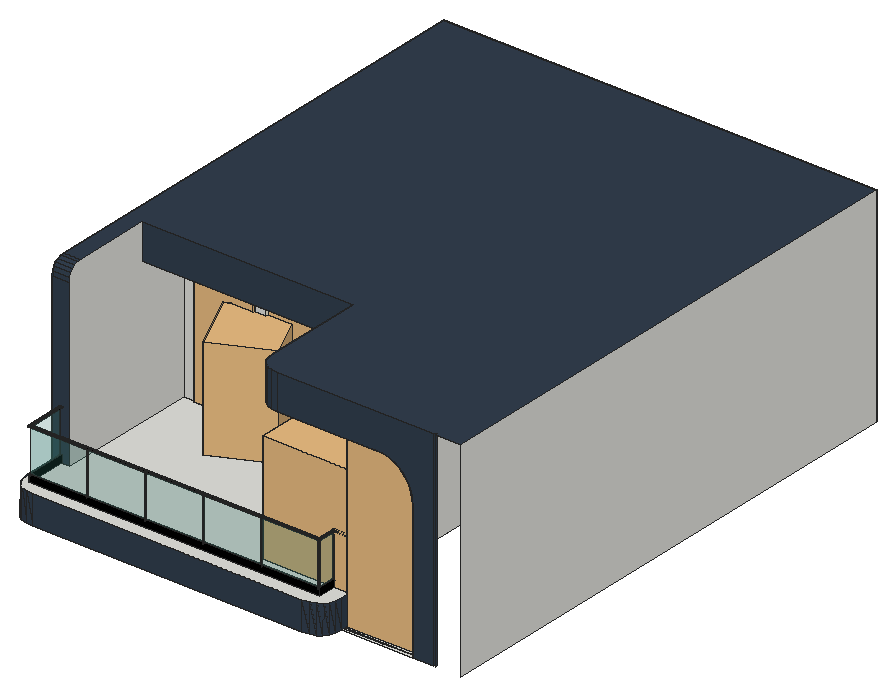
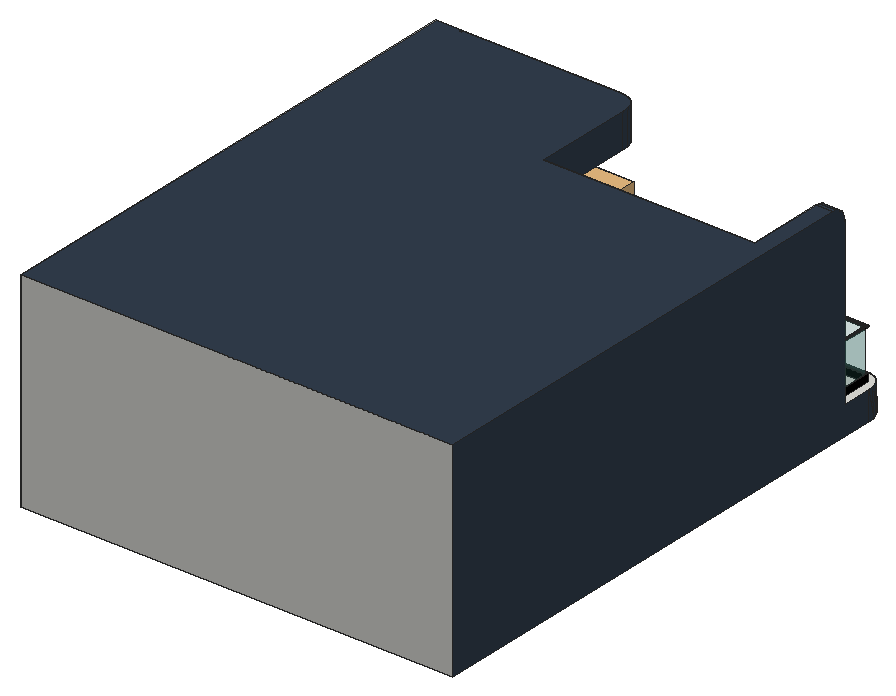
# SketchUp Ruby script. Lengths in inches.
U = 1.inch
M = Sketchup.active_model
def pt(a) = Geom::Point3d.new(a.map { |v| v * U })
def face(e, loops, mat)
  f = e.add_face(loops[0].map { |a| pt(a) })
  loops[1..].each { |l| e.add_face(l.map { |a| pt(a) }).erase! }
  f.material = f.back_material = mat if mat
  f
end
# faces: each face lists its corners as indices into pts; further lists are holes
def faces(e, pts, list, mat = nil) = list.each { |f| face(e, (f[0].is_a?(Array) ? f : [f]).map { |l| l.map { |i| pts[i] } }, mat) }
# xy, xz, yz: faces in a plane at the given z, y or x. An outline is a flat list of corners, or four numbers for a rectangle; further outlines are holes
def ring(l) = l.size == 4 ? [[l[0], l[1]], [l[2], l[1]], [l[2], l[3]], [l[0], l[3]]] : l.each_slice(2).to_a
def flat(e, list, mat, &to3) = list.each { |f| face(e, (f[0].is_a?(Array) ? f : [f]).map { |l| ring(l).map { |u, v| to3.(u, v) } }, mat) }
def xy(e, z, list, mat = nil) = flat(e, list, mat) { |x, y| [x, y, z] }
def xz(e, y, list, mat = nil) = flat(e, list, mat) { |x, z| [x, y, z] }
def yz(e, x, list, mat = nil) = flat(e, list, mat) { |y, z| [x, y, z] }
def lines(e, pts, list) = list.each { |a, b| e.add_line(pt(pts[a]), pt(pts[b])) }
# prism: a flat outline (further loops are holes) pulled along v
def prism(e, loops, v, mat = nil)
  f = face(e, loops, mat); d = Geom::Vector3d.new(v.map { |x| x * U })
  f.pushpull(f.normal.samedirection?(d) ? d.length : -d.length)
end
def box(e, o, s, mat = nil) = prism(e, [[o, [o[0] + s[0], o[1], o[2]], [o[0] + s[0], o[1] + s[1], o[2]], [o[0], o[1] + s[1], o[2]]]], [0, 0, s[2]], mat)
def at(x, y, z, deg = 0) = Geom::Transformation.translation(pt([x, y, z])) * Geom::Transformation.rotation(ORIGIN, Z_AXIS, deg.degrees)
def axes(o, x, y, z) = Geom::Transformation.new([*x, 0, *y, 0, *z, 0, *pt(o).to_a, 1])
def part(name) = M.definitions.add(name)
# library, detail: a bought-in or finely detailed component or shape, given as its bounding box
def library(name, o, s) = part(name).tap { |d| box(d.entities, o, s) }
def detail(e, o, s) = box(e.add_group.entities, o, s)
def put(e, d, t, mat = nil) = e.add_instance(d, t).tap { |i| i.material = mat if mat }
def group(e, t, mat = nil) = e.add_group.tap { |g| g.transformation = t; g.material = mat if mat }.entities
root = M.entities
M.materials.add("0399 AP 9182 LOST BLUE").color = [86, 115, 133]
M.materials.add("0400 AP 7301 PLUTO").color = [50, 63, 78]
M.materials.add("0897 AP 7835 CREAM CARESS").color = [247, 240, 216]
M.materials.add("Glass Railing Color").color = [198, 198, 198]
M.materials.add("Railing Glass").color = [63, 150, 137]
M.materials["Railing Glass"].alpha = 0.13
M.materials.add("[Color M09]").color = [0, 0, 0]
M.materials.add("[Wood Cherry Original]").color = [152, 86, 42]
M.materials.add("ground1").color = [30, 21, 16]
c1 = library("Group45\#2",[-24.46,-60,0],[48.92,120,0.375])
c2 = library("Cay chuoi",[-26.05,-21.66,0],[63.57,52.43,69.02])
c3 = library("door by lz",[5.91,-4.92,0],[35.43,6.61,78.74])
c4 = library("Спалня Венид",[0.07,-0.07,0],[84.71,86.8,39])
c5 = part("Glass Rail Spacer")
box(c5.entities,[-0.5,-0.25,0],[1,0.5,1],"Glass Railing Color")
c6 = part("Group97\#1")
xz(c6.entities,0,[[0.01,0,-0.18,0.02,-0.37,0.09,-0.52,0.21,-0.64,0.37,-0.72,0.54,-0.75,0.74,-0.73,0.93,-0.66,1.12,-0.54,1.27,-0.38,1.39,-0.21,1.47,-0.01,1.5,0.18,1.48,0.37,1.41,0.52,1.29,0.64,1.13,0.72,0.96,0.75,0.76,0.73,0.57,0.66,0.38,0.54,0.23,0.38,0.11,0.21,0.03]],"[Color M09]")
yz(c6.entities,212.09,[[-14.55,0,-14.36,0.03,-14.18,0.11,-14.02,0.23,-13.91,0.38,-13.84,0.57,-13.8125,0.76,-13.84,0.96,-13.92,1.13,-14.04,1.29,-14.2,1.41,-14.38,1.48,-14.57,1.5,-14.77,1.47,-14.95,1.39,-15.1,1.27,-15.22,1.12,-15.29,0.93,-15.3125,0.74,-15.28,0.54,-15.21,0.37,-15.08,0.21,-14.93,0.09,-14.75,0.02]],"[Color M09]")
p = [[-0.18,0,0.02],[-0.18,-27.5,0.02],[-0.37,-27.68,0.09],[-0.37,0,0.09],[200.81,-27.5,0.02],[200.99,-27.68,0.09],
  [200.81,-14.75,0.02],[200.99,-14.93,0.09],[0.01,0,0],[0.01,-27.3,0],[200.61,-27.3,0],[200.61,-14.55,0],
  [0.21,0,0.03],[0.21,-27.11,0.03],[200.42,-27.11,0.03],[200.42,-14.36,0.03],[0.38,0,0.11],[0.38,-26.93,0.11],
  [200.24,-26.93,0.11],[200.24,-14.18,0.11],[212.09,-14.75,0.02],[212.09,-14.93,0.09],[212.09,-14.55,0],[212.09,-14.36,0.03],
  [212.09,-14.18,0.11],[-0.52,-27.83,0.21],[-0.52,0,0.21],[201.15,-27.83,0.21],[201.15,-15.08,0.21],[0.54,0,0.23],
  [0.54,-26.77,0.23],[200.09,-26.77,0.23],[200.09,-14.02,0.23],[212.09,-15.08,0.21],[212.09,-14.02,0.23],[-0.64,-27.96,0.37],
  [-0.64,0,0.37],[201.27,-27.96,0.37],[201.27,-15.21,0.37],[0.66,0,0.38],[0.66,-26.66,0.38],[199.97,-26.66,0.38],
  [199.97,-13.91,0.38],[212.09,-15.21,0.37],[212.09,-13.91,0.38],[-0.72,-28.03,0.54],[-0.72,0,0.54],[201.35,-28.03,0.54],
  [201.35,-15.28,0.54],[0.73,0,0.57],[0.73,-26.59,0.57],[199.9,-26.59,0.57],[199.9,-13.84,0.57],[212.09,-15.28,0.54],
  [212.09,-13.84,0.57],[-0.75,-28.0625,0.74],[-0.75,0,0.74],[201.375,-28.0625,0.74],[201.375,-15.3125,0.74],[212.09,-15.3125,0.74],
  [0.75,0,0.76],[0.75,-26.5625,0.76],[199.875,-26.5625,0.76],[199.875,-13.8125,0.76],[212.09,-13.8125,0.76],[-0.73,-28.04,0.93],
  [-0.73,0,0.93],[201.35,-28.04,0.93],[201.35,-15.29,0.93],[212.09,-15.29,0.93],[0.72,0,0.96],[0.72,-26.59,0.96],
  [199.9,-26.59,0.96],[199.9,-13.84,0.96],[212.09,-13.84,0.96],[-0.66,-27.97,1.12],[-0.66,0,1.12],[201.28,-27.97,1.12],
  [201.28,-15.22,1.12],[212.09,-15.22,1.12],[0.64,0,1.13],[0.64,-26.67,1.13],[199.98,-26.67,1.13],[199.98,-13.92,1.13],
  [212.09,-13.92,1.13],[-0.54,-27.85,1.27],[-0.54,0,1.27],[201.16,-27.85,1.27],[201.16,-15.1,1.27],[0.52,0,1.29],
  [0.52,-26.79,1.29],[200.1,-26.79,1.29],[200.1,-14.04,1.29],[212.09,-15.1,1.27],[212.09,-14.04,1.29],[-0.38,-27.7,1.39],
  [-0.38,0,1.39],[201.01,-27.7,1.39],[201.01,-14.95,1.39],[0.37,0,1.41],[0.37,-26.95,1.41],[200.26,-26.95,1.41],
  [200.26,-14.2,1.41],[212.09,-14.95,1.39],[212.09,-14.2,1.41],[-0.21,-27.52,1.47],[-0.21,0,1.47],[200.83,-27.52,1.47],
  [200.83,-14.77,1.47],[0.18,0,1.48],[0.18,-27.13,1.48],[200.44,-27.13,1.48],[200.44,-14.38,1.48],[212.09,-14.77,1.47],
  [212.09,-14.38,1.48],[-0.01,-27.32,1.5],[-0.01,0,1.5],[200.64,-27.32,1.5],[200.64,-14.57,1.5],[212.09,-14.57,1.5]]
faces(c6.entities,p,[[0,1,2,3],[1,4,5,2],[4,6,7,5],[8,9,1,0],[9,10,4,1],[10,11,6,4],[12,13,9,8],[13,14,10,9],
  [14,15,11,10],[16,17,13,12],[17,18,14,13],[18,19,15,14],[6,20,21,7],[11,22,20,6],[15,23,22,11],[19,24,23,15],
  [3,2,25,26],[2,5,27,25],[5,7,28,27],[29,30,17,16],[30,31,18,17],[31,32,19,18],[7,21,33,28],[32,34,24,19],
  [26,25,35,36],[25,27,37,35],[27,28,38,37],[39,40,30,29],[40,41,31,30],[41,42,32,31],[28,33,43,38],[42,44,34,32],
  [36,35,45,46],[35,37,47,45],[37,38,48,47],[49,50,40,39],[50,51,41,40],[51,52,42,41],[38,43,53,48],[52,54,44,42],
  [46,45,55,56],[45,47,57,55],[47,48,58,57],[48,53,59,58],[60,61,50,49],[61,62,51,50],[62,63,52,51],[63,64,54,52],
  [56,55,65,66],[55,57,67,65],[57,58,68,67],[58,59,69,68],[70,71,61,60],[71,72,62,61],[72,73,63,62],[73,74,64,63],
  [66,65,75,76],[65,67,77,75],[67,68,78,77],[68,69,79,78],[80,81,71,70],[81,82,72,71],[82,83,73,72],[83,84,74,73],
  [76,75,85,86],[75,77,87,85],[77,78,88,87],[89,90,81,80],[90,91,82,81],[91,92,83,82],[78,79,93,88],[92,94,84,83],
  [86,85,95,96],[85,87,97,95],[87,88,98,97],[99,100,90,89],[100,101,91,90],[101,102,92,91],[88,93,103,98],[102,104,94,92],
  [96,95,105,106],[95,97,107,105],[97,98,108,107],[109,110,100,99],[110,111,101,100],[111,112,102,101],[98,103,113,108],[112,114,104,102],
  [106,105,115,116],[105,107,117,115],[107,108,118,117],[116,115,110,109],[115,117,111,110],[117,118,112,111],[108,113,119,118],[118,119,114,112]],"[Color M09]")
c7 = part("Group100\#1")
xy(c7.entities,0,[[-0.5,-27.8125,-0.5,0,0.5,0,0.5,-26.8125],[-0.5,-27.8125,0.5,-26.8125,200.125,-26.8125,201.125,-27.8125],[201.125,-27.8125,200.125,-26.8125,200.125,-14.0625,201.125,-15.0625],[201.125,-15.0625,200.125,-14.0625,212.09,-14.0625,212.09,-15.0625]],"[Color M09]")
xy(c7.entities,4,[[-0.25,-27.5625,0.25,-27.0625,0.25,0,-0.25,0],[-0.25,-27.5625,200.875,-27.5625,200.375,-27.0625,0.25,-27.0625],[200.875,-27.5625,200.875,-14.8125,200.375,-14.3125,200.375,-27.0625],[200.875,-14.8125,212.09,-14.8125,212.09,-14.3125,200.375,-14.3125]],"[Color M09]")
xy(c7.entities,5,[[-0.5,-27.8125,-0.25,-27.5625,-0.25,0,-0.5,0],[-0.5,-27.8125,201.125,-27.8125,200.875,-27.5625,-0.25,-27.5625],[201.125,-27.8125,201.125,-15.0625,200.875,-14.8125,200.875,-27.5625],[0.25,-27.0625,0.5,-26.8125,0.5,0,0.25,0],[0.25,-27.0625,200.375,-27.0625,200.125,-26.8125,0.5,-26.8125],
  [200.375,-27.0625,200.375,-14.3125,200.125,-14.0625,200.125,-26.8125],[201.125,-15.0625,212.09,-15.0625,212.09,-14.8125,200.875,-14.8125],[200.375,-14.3125,212.09,-14.3125,212.09,-14.0625,200.125,-14.0625]],"[Color M09]")
xz(c7.entities,-27.8125,[[-0.5,0,201.125,5]],"[Color M09]")
xz(c7.entities,-27.5625,[[-0.25,4,200.875,5]],"[Color M09]")
xz(c7.entities,-27.0625,[[0.25,4,200.375,5]],"[Color M09]")
xz(c7.entities,-26.8125,[[0.5,0,200.125,5]],"[Color M09]")
xz(c7.entities,-15.0625,[[201.125,0,212.09,5]],"[Color M09]")
xz(c7.entities,-14.8125,[[200.875,4,212.09,5]],"[Color M09]")
xz(c7.entities,-14.3125,[[200.375,4,212.09,5]],"[Color M09]")
xz(c7.entities,-14.0625,[[200.125,0,212.09,5]],"[Color M09]")
xz(c7.entities,0,[[-0.5,0,-0.5,5,-0.25,5,-0.25,4,0.25,4,0.25,5,0.5,5,0.5,0]],"[Color M09]")
yz(c7.entities,-0.5,[[-27.8125,0,0,5]],"[Color M09]")
yz(c7.entities,-0.25,[[-27.5625,4,0,5]],"[Color M09]")
yz(c7.entities,0.25,[[-27.0625,4,0,5]],"[Color M09]")
yz(c7.entities,0.5,[[-26.8125,0,0,5]],"[Color M09]")
yz(c7.entities,200.125,[[-26.8125,0,-14.0625,5]],"[Color M09]")
yz(c7.entities,200.375,[[-27.0625,4,-14.3125,5]],"[Color M09]")
yz(c7.entities,200.875,[[-27.5625,4,-14.8125,5]],"[Color M09]")
yz(c7.entities,201.125,[[-27.8125,0,-15.0625,5]],"[Color M09]")
yz(c7.entities,212.09,[[-15.0625,0,-14.0625,0,-14.0625,5,-14.3125,5,-14.3125,4,-14.8125,4,-14.8125,5,-15.0625,5]],"[Color M09]")
c8 = part("Group101\#2")
box(c8.entities,[-0.1875,0,0],[0.375,25.5625,30],"Railing Glass")
c9 = part("Group102\#2")
box(c9.entities,[-0.1875,0,0],[0.375,39.03,30],"Railing Glass")
c10 = part("Group103\#2")
box(c10.entities,[-0.1875,0,0],[0.375,39.02,30],"Railing Glass")
c11 = part("Group104\#2")
box(c11.entities,[-0.1875,0,0],[0.375,39.02,30],"Railing Glass")
c12 = part("Group105\#2")
box(c12.entities,[-0.1875,0,0],[0.375,39.03,30],"Railing Glass")
c13 = part("Group106\#2")
box(c13.entities,[-0.1875,0,0],[0.375,39.03,30],"Railing Glass")
c14 = part("Group107\#1")
box(c14.entities,[-0.1875,0,0],[0.375,11.25,30],"Railing Glass")
c15 = part("Group108\#1")
box(c15.entities,[-0.1875,0,0],[0.375,9.71,30],"Railing Glass")
c16 = part("Glass Railing\#1")
put(c16.entities,c5,at(0,0,4,-90))
put(c16.entities,c5,at(0,-26.5625,4,-90))
put(c16.entities,c5,at(0.25,-26.8125,4))
put(c16.entities,c5,at(40.28,-26.8125,4))
put(c16.entities,c5,at(80.3,-26.8125,4))
put(c16.entities,c5,at(120.32,-26.8125,4))
put(c16.entities,c5,at(160.35,-26.8125,4))
put(c16.entities,c5,at(200.375,-26.8125,4))
put(c16.entities,c5,at(200.625,-26.5625,4,90))
put(c16.entities,c5,at(200.625,-14.3125,4,90))
put(c16.entities,c5,at(200.875,-14.0625,4))
put(c16.entities,c5,at(211.59,-14.0625,4))
put(c16.entities,c6,at(0,0.5,34),"Glass Railing Color")
put(c16.entities,c7,at(0,0.5,0),"Glass Railing Color")
put(c16.entities,c8,at(0,-0.5,4,180),"Railing Glass")
put(c16.entities,c9,at(0.75,-26.8125,4,-90),"Railing Glass")
put(c16.entities,c10,at(40.78,-26.8125,4,-90),"Railing Glass")
put(c16.entities,c11,at(80.8,-26.8125,4,-90),"Railing Glass")
put(c16.entities,c12,at(120.82,-26.8125,4,-90),"Railing Glass")
put(c16.entities,c13,at(160.85,-26.8125,4,-90),"Railing Glass")
put(c16.entities,c14,at(200.625,-26.0625,4),"Railing Glass")
put(c16.entities,c15,at(201.375,-14.0625,4,-90),"Railing Glass")
c17 = library("cay+chuoi",[26.89,19.66,0.52],[41.96,45.65,69.71])
c18 = library("Sliding windows",[297.42,-0.89,0.35],[194.88,8.85,122.84])
c19 = library("шторы раздвинутые\#1",[23.6875,-79.1875,1.01],[68.3125,79.67,5.17])
c20 = part("Group\#7")
xy(c20.entities,0,[[1.02,0,0.76,0.03,0.51,0.14,0.3,0.3,0.14,0.51,0.03,0.76,0,1.02,0.03,1.28,0.14,1.53,0.3,1.74,0.51,1.9,0.76,2.01,1.02,2.04,1.28,2.01,1.53,1.9,1.74,1.74,1.9,1.53,2.01,1.28,2.04,1.02,2.01,0.76,1.9,0.51,1.74,0.3,1.53,0.14,1.28,0.03]])
c21 = part("Group\#18")
detail(c21.entities,[3.14,3.14,12.38],[2.62,2.62,0.48])
put(c21.entities,c20,at(3.43,3.43,12.51))
c22 = part("Group\#9")
detail(c22.entities,[3.14,3.14,12.38],[2.62,2.62,0.48])
put(c22.entities,c20,at(3.43,3.43,12.51))
xy(root,134,[[543.54,244.875,592.46,246.8125],[543.54,247.8125,592.46,249.875]])
xy(root,134,[[341.36,229.875,336.65,230.29,332.8,231.54,329.81,233.625,327.67,236.54,326.38,240.29,325.96,244.875,543.54,244.875,543.11,240.29,541.83,236.54,539.69,233.625,536.7,231.54,532.84,230.29,528.14,229.875]],"0399 AP 9182 LOST BLUE")
xy(root,154,[[341.36,229.875,528.14,229.875,532.84,230.3,536.7,231.59,539.69,233.73,541.83,236.72,543.11,240.57,543.54,245.28,543.54,364.875,386.96,364.875,386.96,371.625,345.96,371.625,345.96,364.875,337.96,364.875,337.96,266.125,325.96,266.125,325.96,245.28,326.38,240.57,327.67,236.72,329.81,233.73,332.8,231.59,336.65,230.3],[394.96,372.875,523.33,484.875]])
xy(root,162,[[394.96,364.875,523.33,372.875]])
xy(root,244.125,[[345.96,364.875,386.96,371.625]])
xy(root,244.125,[[[394.96,364.875,523.33,484.875],[409.16,379.08,509.125,470.67]],[410.16,380.08,508.125,469.67]],"0897 AP 7835 CREAM CARESS")
xy(root,254,[[499.44,244.875,494.71,245.31,490.84,246.6,487.83,248.75,485.68,251.76,484.39,255.63,483.96,260.36,483.96,328.875,337.96,328.875,337.96,345.875,500.96,345.875,500.96,278.31,501.4,273.42,502.77,269.3,505.11,266.03,508.38,263.69,512.5,262.32,517.4,261.875,543.54,261.875,543.54,244.875],[543.54,244.875,568,246.8125],[543.54,247.8125,568,249.875],[517.44,262.875,512.71,263.31,508.84,264.6,505.83,266.75,503.68,269.76,502.39,273.63,501.96,278.36,501.96,346.875,337.96,346.875,337.96,364.875,543.54,364.875,543.54,262.875]])
xy(root,278,[[499.44,244.875,607.46,244.875,607.46,245.875,608.46,245.875,608.46,244.875,625.96,244.875,625.96,604.875,325.96,604.875,325.96,276.16,337.96,276.16,337.96,328.875,483.96,328.875,483.96,260.36,484.39,255.63,485.68,251.76,487.83,248.75,490.84,246.6,494.71,245.31]],"0400 AP 7301 PLUTO")
xz(root,229.875,[[341.36,134,528.14,154]],"0400 AP 7301 PLUTO")
xz(root,244.875,[[592.46,134,607.46,134,607.46,278,499.44,278,499.44,254,568,254,571.19,253.79,574.33,253.17,577.36,252.14,580.23,250.72,582.89,248.95,585.29,246.84,587.4,244.43,589.18,241.77,590.59,238.9,591.62,235.87,592.25,232.73,592.46,229.54]],"0400 AP 7301 PLUTO")
xz(root,266.125,[[325.96,154,337.96,267.96]],"0400 AP 7301 PLUTO")
xz(root,328.875,[[337.96,254,483.96,278]],"0400 AP 7301 PLUTO")
xz(root,364.875,[[[337.96,154,345.96,154,345.96,244.125,386.96,244.125,386.96,154,543.54,154,543.54,254,337.96,254],[394.96,162,523.33,244.125]]])
xz(root,371.625,[[345.96,154,386.96,244.125]])
xz(root,372.875,[[394.96,154,523.33,162]])
xz(root,484.875,[[394.96,154,523.33,244.125]],"0897 AP 7835 CREAM CARESS")
xz(root,604.875,[[325.96,134,625.96,278]])
yz(root,325.96,[[244.875,134,245.28,154,266.125,154,266.125,267.96,266.4,271.03,267.24,273.54,268.63,275.49,270.59,276.88,273.1,277.72,276.16,278,604.875,278,604.875,134]],"0400 AP 7301 PLUTO")
yz(root,337.96,[[266.125,154,364.875,154,364.875,254,328.875,254,328.875,278,276.16,278,273.1,277.72,270.59,276.88,268.63,275.49,267.24,273.54,266.4,271.03,266.125,267.96]])
yz(root,345.96,[[364.875,154,371.625,244.125]])
yz(root,386.96,[[364.875,154,371.625,244.125]])
yz(root,394.96,[[372.875,154,484.875,154,484.875,244.125,364.875,244.125,364.875,162,372.875,162]],"0897 AP 7835 CREAM CARESS")
yz(root,483.96,[[260.36,254,328.875,278]],"0400 AP 7301 PLUTO")
yz(root,523.33,[[372.875,154,372.875,162,364.875,162,364.875,244.125,484.875,244.125,484.875,154]],"0897 AP 7835 CREAM CARESS")
yz(root,543.54,[[249.875,154,364.875,254]])
yz(root,543.54,[[244.875,134,249.875,134,249.875,154,245.28,154]],"0400 AP 7301 PLUTO")
yz(root,592.46,[[244.875,134,246.8125,229.54],[247.8125,134,249.875,229.54]])
yz(root,607.46,[[244.875,134,245.875,278]],"0400 AP 7301 PLUTO")
yz(root,608.46,[[244.875,134,245.875,278]],"0400 AP 7301 PLUTO")
yz(root,625.96,[[244.875,134,604.875,278]])
p = [[341.36,229.875,134],[341.36,229.875,154],[336.65,230.3,154],[336.65,230.29,134],[532.84,230.29,134],[532.84,230.3,154],
  [528.14,229.875,154],[528.14,229.875,134],[332.8,231.54,134],[332.8,231.59,154],[536.7,231.54,134],[536.7,231.59,154],
  [329.81,233.73,154],[329.81,233.625,134],[539.69,233.625,134],[539.69,233.73,154],[327.67,236.72,154],[327.67,236.54,134],
  [541.83,236.54,134],[541.83,236.72,154],[326.38,240.57,154],[326.38,240.29,134],[543.11,240.29,134],[543.11,240.57,154],
  [325.96,245.28,154],[325.96,244.875,134],[543.54,244.875,134],[543.54,245.28,154],[592.25,244.875,232.73],[592.25,246.8125,232.73],
  [592.46,246.8125,229.54],[592.46,244.875,229.54],[592.46,249.875,229.54],[592.46,247.8125,229.54],[592.25,247.8125,232.73],[592.25,249.875,232.73],
  [591.62,244.875,235.87],[591.62,246.8125,235.87],[591.62,247.8125,235.87],[591.62,249.875,235.87],[590.59,244.875,238.9],[590.59,246.8125,238.9],
  [590.59,247.8125,238.9],[590.59,249.875,238.9],[589.18,244.875,241.77],[589.18,246.8125,241.77],[589.18,247.8125,241.77],[589.18,249.875,241.77],
  [587.4,244.875,244.43],[587.4,246.8125,244.43],[587.4,247.8125,244.43],[587.4,249.875,244.43],[585.29,244.875,246.84],[585.29,246.8125,246.84],
  [585.29,247.8125,246.84],[585.29,249.875,246.84],[582.89,244.875,248.95],[582.89,246.8125,248.95],[582.89,247.8125,248.95],[582.89,249.875,248.95],
  [580.23,244.875,250.72],[580.23,246.8125,250.72],[580.23,247.8125,250.72],[580.23,249.875,250.72],[577.36,244.875,252.14],[577.36,246.8125,252.14],
  [577.36,247.8125,252.14],[577.36,249.875,252.14],[574.33,244.875,253.17],[574.33,246.8125,253.17],[574.33,247.8125,253.17],[574.33,249.875,253.17],
  [571.19,244.875,253.79],[571.19,246.8125,253.79],[571.19,247.8125,253.79],[571.19,249.875,253.79],[568,244.875,254],[568,246.8125,254],
  [568,247.8125,254],[568,249.875,254],[494.71,245.31,278],[494.71,245.31,254],[499.44,244.875,254],[499.44,244.875,278],
  [490.84,246.6,278],[490.84,246.6,254],[487.83,248.75,278],[487.83,248.75,254],[485.68,251.76,278],[485.68,251.76,254],
  [484.39,255.63,278],[484.39,255.63,254],[483.96,260.36,278],[483.96,260.36,254],[325.96,266.125,267.96],[337.96,266.125,267.96],
  [337.96,266.4,271.03],[325.96,266.4,271.03],[337.96,267.24,273.54],[325.96,267.24,273.54],[337.96,268.63,275.49],[325.96,268.63,275.49],
  [337.96,270.59,276.88],[325.96,270.59,276.88],[337.96,273.1,277.72],[325.96,273.1,277.72],[337.96,276.16,278],[325.96,276.16,278],
  [593.33,247.8125,134],[592.46,247.8125,134],[593.33,246.8125,134],[592.46,246.8125,134]]
faces(root,p,[[0,1,2],[3,0,2],[4,5,6],[7,4,6],[8,3,9],[3,2,9],[10,11,5],[4,10,5],
  [8,9,12],[13,8,12],[10,14,11],[14,15,11],[13,12,16],[17,13,16],[14,18,15],[18,19,15],
  [17,16,20],[21,17,20],[18,22,19],[22,23,19],[21,20,24],[25,21,24],[22,26,23],[26,27,23],
  [80,81,82,83],[84,85,81,80],[86,87,85,84],[88,89,87,86],[90,91,89,88],[92,93,91,90],[94,95,96,97],[97,96,98,99],
  [99,98,100,101],[101,100,102,103],[103,102,104,105],[105,104,106,107]],"0400 AP 7301 PLUTO")
faces(root,p,[[28,29,30,31],[32,33,34,35],[36,37,29,28],[35,34,38,39],[40,41,37,36],[39,38,42,43],[44,45,41,40],[43,42,46,47],
  [48,49,45,44],[47,46,50,51],[52,53,49,48],[51,50,54,55],[56,57,53,52],[55,54,58,59],[60,61,57,56],[59,58,62,63],
  [64,65,61,60],[63,62,66,67],[68,69,65,64],[67,66,70,71],[72,73,69,68],[71,70,74,75],[76,77,73,72],[75,74,78,79]])
lines(root,p,[[108,109],[110,111]])
put(root,c1,axes([568,249.875,194],[1,0,0],[0,0,1],[0,-1,0]),"[Wood Cherry Original]")
g1 = group(root,at(543.54,246.8125,134))
xy(g1,0,[[0,0,48.91,1]])
xy(g1,120,[[0,0,24.46,1]])
yz(g1,48.91,[[0,0,1,95.54]])
p = [[48.71,0,98.73],[48.71,1,98.73],[48.91,1,95.54],[48.91,0,95.54],[48.08,0,101.87],[48.08,1,101.87],
  [47.05,0,104.9],[47.05,1,104.9],[45.64,0,107.77],[45.64,1,107.77],[43.86,0,110.43],[43.86,1,110.43],
  [41.75,0,112.84],[41.75,1,112.84],[39.35,0,114.95],[39.35,1,114.95],[36.6875,0,116.72],[36.6875,1,116.72],
  [33.82,0,118.14],[33.82,1,118.14],[30.79,0,119.17],[30.79,1,119.17],[27.65,0,119.79],[27.65,1,119.79],
  [24.46,0,120],[24.46,1,120]]
faces(g1,p,[[0,1,2,3],[4,5,1,0],[6,7,5,4],[8,9,7,6],[10,11,9,8],[12,13,11,10],[14,15,13,12],[16,17,15,14],
  [18,19,17,16],[20,21,19,18],[22,23,21,20],[24,25,23,22]])
put(root,c2,axes([512.3125,275.34,154],[1.11,0,0],[0,1.11,0],[0,0,1.11]),"ground1")
put(root,c3,axes([339.11,368.91,154],[1.15711,0,0],[0,1,0],[0,0,1.14459]))
put(root,c4,at(481.42,395.63,154,90))
put(root,c16,at(331.96,266.125,154))
put(root,c17,at(370.64,291.7,154,24.9))
put(root,c18,axes([199.04,366.94,161.76],[0.65873,0,0],[0,0.54,0],[0,0,0.66858]))
put(root,c19,axes([347.58,380.45,243.65],[2,0,0],[0,0,1],[0,-1,0]))
g2 = group(root,at(444.72,483.87,190),"[Color M09]")
xy(g2,0,[[0,0,33.4375,1]])
xy(g2,0.96,[[0.86,0,32.58,0.125]])
xy(g2,37.75,[[0.86,0,32.58,0.125]])
xy(g2,38.71,[[0,0,33.4375,1]])
xz(g2,0,[[[0,0,33.4375,38.71],[0.86,0.96,32.58,37.75]]])
xz(g2,0.125,[[0.86,0.96,32.58,37.75]])
xz(g2,1,[[0,0,33.4375,38.71]])
yz(g2,0,[[0,0,1,38.71]])
yz(g2,0.86,[[0,0.96,0.125,37.75]])
yz(g2,32.58,[[0,0.96,0.125,37.75]])
yz(g2,33.4375,[[0,0,1,38.71]])
put(root,c21,at(400.04,384.76,231.27))
put(root,c21,at(400.04,422.26,231.27))
put(root,c21,at(400.04,470.82,231.27))
put(root,c21,at(510.92,384.76,231.27))
put(root,c21,at(510.92,422.26,231.27))
put(root,c21,at(510.92,470.82,231.27))
put(root,c21,at(455.85,384.76,231.27))
put(root,c21,at(455.85,470.82,231.27))
g3 = group(root,at(409.16,379.08,244.125))
xy(g3,0,[[[0,0,99.96,91.59],[1,1,98.96,90.59]]])
put(root,c22,at(519.09,270.65,241.14))
g4 = group(root,at(519.09,294.65,241.14))
detail(g4,[3.14,3.14,12.38],[2.62,2.62,0.48])
put(g4,c20,at(3.43,3.43,12.51))
g5 = group(root,at(519.09,318.65,241.14))
detail(g5,[3.14,3.14,12.38],[2.62,2.62,0.48])
put(g5,c20,at(3.43,3.43,12.51))
g6 = group(root,at(519.09,342.65,241.14))
detail(g6,[3.14,3.14,12.38],[2.62,2.62,0.48])
put(g6,c20,at(3.43,3.43,12.51))
g7 = group(root,at(488.55,347.36,241.14))
detail(g7,[3.14,3.14,12.38],[2.62,2.62,0.48])
put(g7,c20,at(3.43,3.43,12.51))
put(root,c21,at(440.55,347.36,241.14))
g8 = group(root,at(392.55,347.36,241.14))
detail(g8,[3.14,3.14,12.38],[2.62,2.62,0.48])
put(g8,c20,at(3.43,3.43,12.51))
g9 = group(root,at(344.55,351.95,241.14))
detail(g9,[3.14,3.14,12.38],[2.62,2.62,0.48])
put(g9,c20,at(3.43,3.43,12.51))
g10 = group(root,at(337.96,261.875,254))
xy(g10,0,[[179.44,0,174.55,0.44,170.42,1.82,167.15,4.15,164.82,7.42,163.44,11.55,163,16.44,163,84,0,84,0,85,164,85,164,16.49,164.43,11.75,165.72,7.88,167.87,4.87,170.88,2.72,174.75,1.43,179.49,1,205.59,1,205.59,0]])
